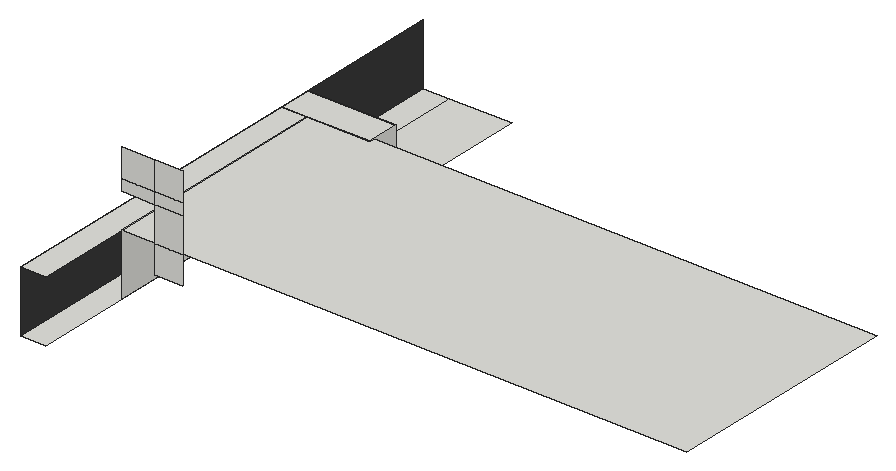
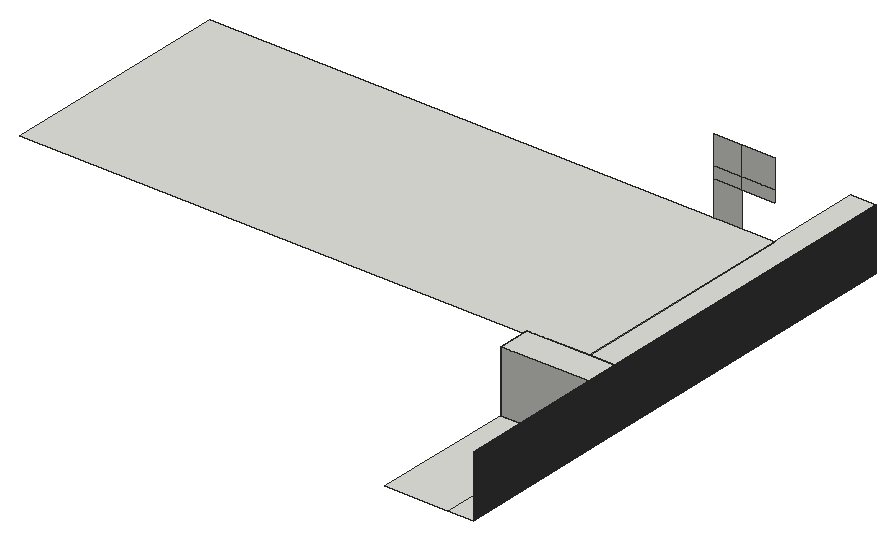
# SketchUp Ruby script. Lengths in inches.
U = 1.inch
M = Sketchup.active_model
def pt(a) = Geom::Point3d.new(a.map { |v| v * U })
def face(e, loops, mat)
  f = e.add_face(loops[0].map { |a| pt(a) })
  loops[1..].each { |l| e.add_face(l.map { |a| pt(a) }).erase! }
  f.material = f.back_material = mat if mat
  f
end
# faces: each face lists its corners as indices into pts; further lists are holes
def faces(e, pts, list, mat = nil) = list.each { |f| face(e, (f[0].is_a?(Array) ? f : [f]).map { |l| l.map { |i| pts[i] } }, mat) }
# xy, xz, yz: faces in a plane at the given z, y or x. An outline is a flat list of corners, or four numbers for a rectangle; further outlines are holes
def ring(l) = l.size == 4 ? [[l[0], l[1]], [l[2], l[1]], [l[2], l[3]], [l[0], l[3]]] : l.each_slice(2).to_a
def flat(e, list, mat, &to3) = list.each { |f| face(e, (f[0].is_a?(Array) ? f : [f]).map { |l| ring(l).map { |u, v| to3.(u, v) } }, mat) }
def xy(e, z, list, mat = nil) = flat(e, list, mat) { |x, y| [x, y, z] }
def xz(e, y, list, mat = nil) = flat(e, list, mat) { |x, z| [x, y, z] }
def yz(e, x, list, mat = nil) = flat(e, list, mat) { |y, z| [x, y, z] }
def lines(e, pts, list) = list.each { |a, b| e.add_line(pt(pts[a]), pt(pts[b])) }
# prism: a flat outline (further loops are holes) pulled along v
def prism(e, loops, v, mat = nil)
  f = face(e, loops, mat); d = Geom::Vector3d.new(v.map { |x| x * U })
  f.pushpull(f.normal.samedirection?(d) ? d.length : -d.length)
end
def box(e, o, s, mat = nil) = prism(e, [[o, [o[0] + s[0], o[1], o[2]], [o[0] + s[0], o[1] + s[1], o[2]], [o[0], o[1] + s[1], o[2]]]], [0, 0, s[2]], mat)
def at(x, y, z, deg = 0) = Geom::Transformation.translation(pt([x, y, z])) * Geom::Transformation.rotation(ORIGIN, Z_AXIS, deg.degrees)
def axes(o, x, y, z) = Geom::Transformation.new([*x, 0, *y, 0, *z, 0, *pt(o).to_a, 1])
def part(name) = M.definitions.add(name)
# library, detail: a bought-in or finely detailed component or shape, given as its bounding box
def library(name, o, s) = part(name).tap { |d| box(d.entities, o, s) }
def detail(e, o, s) = box(e.add_group.entities, o, s)
def put(e, d, t, mat = nil) = e.add_instance(d, t).tap { |i| i.material = mat if mat }
def group(e, t, mat = nil) = e.add_group.tap { |g| g.transformation = t; g.material = mat if mat }.entities
root = M.entities
M.materials.add("[Color M07]").color = [58, 58, 58]
xy(root,240.47,[[2236.57,505.3125,2240.94,561.375],[2236.57,561.375,2240.94,567.01],[2240.94,561.375,2251.71,567.01],[2236.57,567.01,2240.94,591.8125],[2240.94,567.01,2251.71,591.8125]])
xy(root,251.0625,[[2236.57,505.3125,2240.94,561.375],[2240.94,521.5625,2240.94,561.375,2251.71,561.375,2251.71,562.32,2337.96,562.32,2337.96,521.5625],[2236.57,561.375,2251.71,567.01]])
xz(root,521.5625,[[2246.66,246.25,2251.48,251.0625],[2246.66,251.0625,2251.48,257.0625],[2240.94,257.0625,2246.66,258.95],[2246.66,257.0625,2251.48,258.95],[2240.94,258.95,2246.66,263.89],
  [2246.66,258.95,2251.48,263.89]])
xz(root,561.375,[[2236.57,240.47,2240.94,251.0625],[2240.94,240.47,2251.71,251.0625]])
xz(root,567.01,[[2236.57,240.47,2251.71,251.0625]])
yz(root,2236.57,[[505.3125,240.47,561.375,251.0625],[561.375,240.47,567.01,251.0625],[567.01,240.47,591.8125,251.0625]],"[Color M07]")
yz(root,2240.94,[[521.5625,240.47,561.375,251.0625]])
yz(root,2251.71,[[561.375,240.47,567.01,251.0625]])
